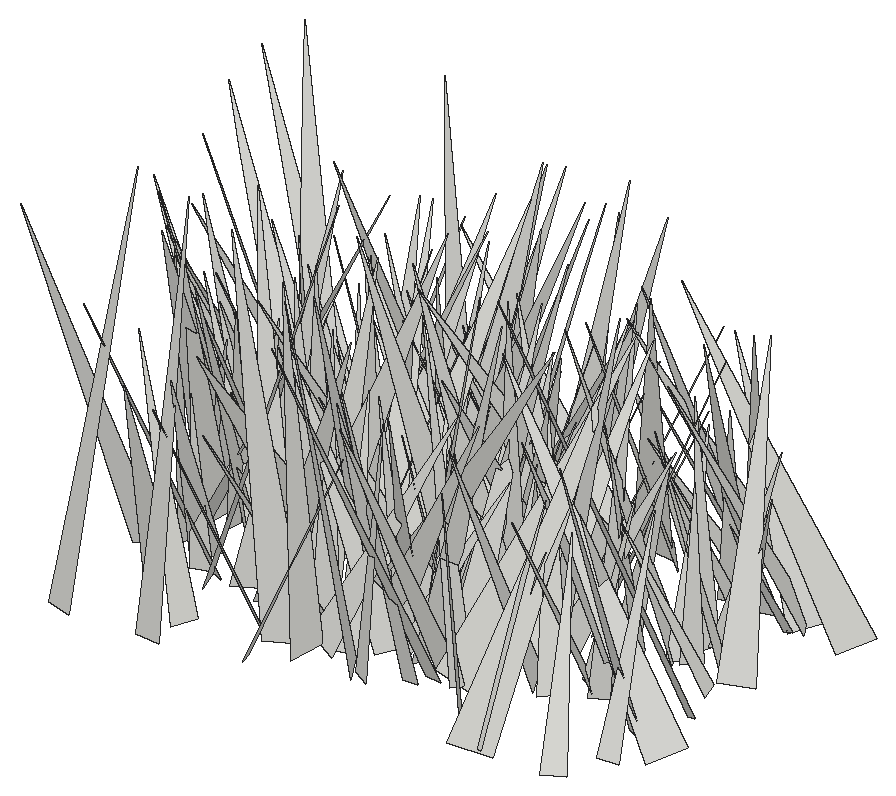
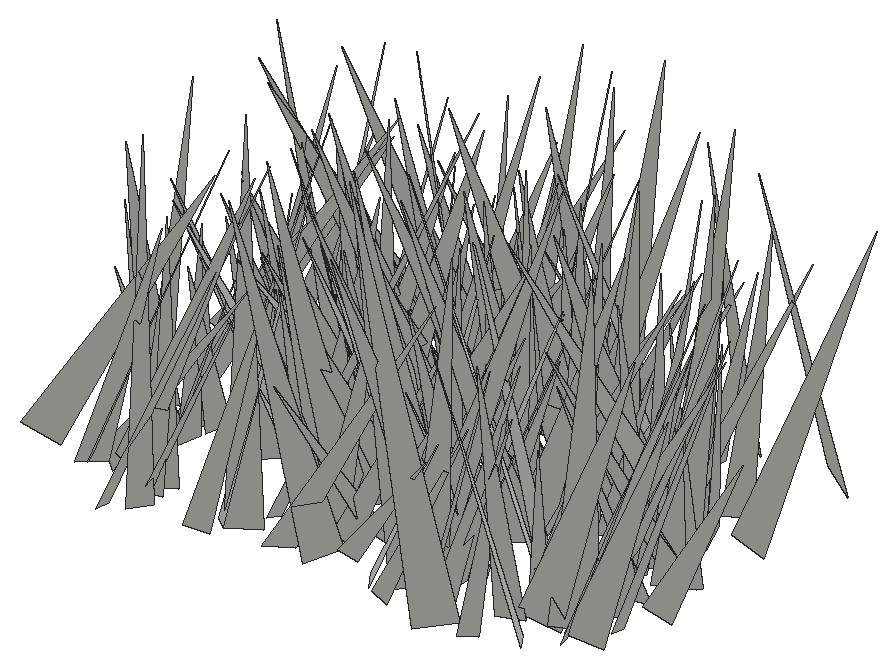
# SketchUp Ruby script. Lengths in inches.
U = 1.inch
M = Sketchup.active_model
def pt(a) = Geom::Point3d.new(a.map { |v| v * U })
def face(e, loops, mat)
  f = e.add_face(loops[0].map { |a| pt(a) })
  loops[1..].each { |l| e.add_face(l.map { |a| pt(a) }).erase! }
  f.material = f.back_material = mat if mat
  f
end
# faces: each face lists its corners as indices into pts; further lists are holes
def faces(e, pts, list, mat = nil) = list.each { |f| face(e, (f[0].is_a?(Array) ? f : [f]).map { |l| l.map { |i| pts[i] } }, mat) }
# xy, xz, yz: faces in a plane at the given z, y or x. An outline is a flat list of corners, or four numbers for a rectangle; further outlines are holes
def ring(l) = l.size == 4 ? [[l[0], l[1]], [l[2], l[1]], [l[2], l[3]], [l[0], l[3]]] : l.each_slice(2).to_a
def flat(e, list, mat, &to3) = list.each { |f| face(e, (f[0].is_a?(Array) ? f : [f]).map { |l| ring(l).map { |u, v| to3.(u, v) } }, mat) }
def xy(e, z, list, mat = nil) = flat(e, list, mat) { |x, y| [x, y, z] }
def xz(e, y, list, mat = nil) = flat(e, list, mat) { |x, z| [x, y, z] }
def yz(e, x, list, mat = nil) = flat(e, list, mat) { |y, z| [x, y, z] }
def lines(e, pts, list) = list.each { |a, b| e.add_line(pt(pts[a]), pt(pts[b])) }
# prism: a flat outline (further loops are holes) pulled along v
def prism(e, loops, v, mat = nil)
  f = face(e, loops, mat); d = Geom::Vector3d.new(v.map { |x| x * U })
  f.pushpull(f.normal.samedirection?(d) ? d.length : -d.length)
end
def box(e, o, s, mat = nil) = prism(e, [[o, [o[0] + s[0], o[1], o[2]], [o[0] + s[0], o[1] + s[1], o[2]], [o[0], o[1] + s[1], o[2]]]], [0, 0, s[2]], mat)
def at(x, y, z, deg = 0) = Geom::Transformation.translation(pt([x, y, z])) * Geom::Transformation.rotation(ORIGIN, Z_AXIS, deg.degrees)
def axes(o, x, y, z) = Geom::Transformation.new([*x, 0, *y, 0, *z, 0, *pt(o).to_a, 1])
def part(name) = M.definitions.add(name)
# library, detail: a bought-in or finely detailed component or shape, given as its bounding box
def library(name, o, s) = part(name).tap { |d| box(d.entities, o, s) }
def detail(e, o, s) = box(e.add_group.entities, o, s)
def put(e, d, t, mat = nil) = e.add_instance(d, t).tap { |i| i.material = mat if mat }
def group(e, t, mat = nil) = e.add_group.tap { |g| g.transformation = t; g.material = mat if mat }.entities
root = M.entities
c1 = part("fur_instance\#9")
p = [[0.8125,0,1.79],[0.67,-0.02,1.48],[0,-0.11,0],[0,0.11,0]]
faces(c1.entities,p,[[0,1,2,3]])
put(root,c1,axes([458.25,101.48,-21.86],[3.84252,-3.67557,0.42443],[-3.56655,-3.84235,-0.9854],[-0.98471,-0.42605,5.2253]))
put(root,c1,axes([461.14,97.17,-21.66],[2.8075,7.47142,1.47372],[7.21104,-3.11318,2.04573],[-2.44844,-0.60171,7.71486]))
put(root,c1,axes([467.92,100.34,-21.86],[-6.16765,-3.82155,1.90605],[-3.98751,6.35208,-0.16723],[1.52874,1.15063,7.2537]))
put(root,c1,axes([473.27,99.74,-21.86],[-3.53133,-2.30027,1.49102],[-2.55807,3.63918,-0.44418],[0.98523,1.20406,4.19097]))
put(root,c1,axes([463.6,100.56,-21.86],[-3.04212,-3.44962,0.11938],[-3.35963,2.92271,-1.15727],[-0.79185,0.85236,4.45141]))
put(root,c1,axes([457.1,97.23,-21.86],[3.59561,7.30217,1.1805],[7.09033,-3.77639,1.76345],[-2.10771,-0.24675,7.94609]))
put(root,c1,axes([464.9,100.28,-21.86],[1.59006,-7.38899,3.46765],[-7.94346,-2.21328,-1.07372],[-1.87702,3.10714,7.48148]))
put(root,c1,axes([461.2,99.19,-21.86],[-5.26641,1.25593,0.32091],[1.22212,5.2582,-0.5227],[0.43216,0.43524,5.3888]))
put(root,c1,axes([478.27,98.73,-21.86],[-2.52047,3.62206,0.22803],[3.61381,2.53037,-0.24846],[0.33426,-0.04477,4.40572]))
put(root,c1,axes([464.5,98.53,-21.86],[4.05537,2.07279,0.17475],[1.9711,-3.95155,1.12829],[-0.66463,0.92835,4.41242]))
put(root,c1,axes([465.9,100.24,-21.86],[-6.94561,0.7265,2.56424],[0.79665,7.39636,0.06233],[2.54332,-0.33278,6.98322]))
put(root,c1,axes([470.83,101.21,-21.66],[-3.56669,-5.90918,0.59479],[-5.71236,3.22345,-2.22975],[-1.62517,1.63841,6.53207]))
put(root,c1,axes([474.76,98.625,-21.86],[1.79845,4.31058,0.12569],[4.2592,-1.79684,0.67963],[-0.67534,0.14702,4.621]))
put(root,c1,axes([470.71,102.27,-21.86],[-0.3519,-5.66898,0.64957],[-5.59847,0.21723,-1.13712],[-1.1029,0.70611,5.5649]))
put(root,c1,axes([468.54,99.99,-21.86],[2.39277,4.07076,1.54907],[4.21231,-2.6123,0.35825],[-1.10775,-1.14055,4.7083]))
put(root,c1,axes([466.13,101.58,-21.86],[-1.49578,-4.28811,0.26565],[-3.87905,1.22698,-2.03551],[-1.84701,0.89578,4.0598]))
put(root,c1,axes([474.94,104.88,-21.86],[-3.72735,-5.65721,0.3773],[-4.71825,3.34531,3.54775],[3.14396,-1.68653,5.77153]))
put(root,c1,axes([470.11,100.81,-21.86],[-2.85535,-4.62994,1.75531],[-4.89429,2.33192,-1.81068],[-0.75056,2.40755,5.12941]))
put(root,c1,axes([458.92,103.32,-21.86],[4.17409,-3.35782,0.27535],[-3.2273,-4.11088,-1.20788],[-0.96712,-0.77425,5.2191]))
put(root,c1,axes([467.72,102.88,-21.86],[0.67121,-5.58126,0.90748],[-5.6399,-0.72653,-0.2969],[-0.40679,0.86382,5.61363]))
put(root,c1,axes([466.71,103.46,-21.86],[-1.5232,-7.73744,1.34983],[-7.81047,1.63722,0.57115],[0.82858,1.20901,7.86523]))
put(root,c1,axes([459.89,102.59,-21.86],[-3.27123,-4.88451,0.3113],[-4.82797,3.15879,-1.17003],[-0.80376,0.90546,5.76111]))
put(root,c1,axes([462.75,102.37,-21.86],[5.42547,-4.53511,0.52895],[-4.56014,-5.3411,0.98008],[0.2284,1.09004,7.00303]))
put(root,c1,axes([467.49,104.29,-21.66],[-1.30326,-6.4856,0.41929],[-6.05179,1.36694,2.33336],[2.36951,-0.07596,6.19006]))
put(root,c1,axes([473.47,103.78,-21.86],[-5.10979,-2.8974,1.28802],[-2.4355,5.15064,1.92434],[2.03034,-1.11347,5.54994]))
put(root,c1,axes([478.84,102.74,-21.86],[-2.84226,-5.05917,1.08036],[-5.16298,2.85167,-0.22901],[0.32566,1.05526,5.79838]))
put(root,c1,axes([474.01,100.5,-21.86],[0.88242,4.55252,0.64978],[4.54635,-0.76413,-0.82042],[0.6916,-0.78549,4.5641]))
put(root,c1,axes([462.64,105.77,-21.66],[6.08431,-4.17162,0.61258],[-3.3903,-5.47976,-3.64343],[-2.50671,-2.71408,6.41457]))
put(root,c1,axes([465.93,100.97,-21.86],[1.55014,5.60518,1.20615],[5.3228,-0.94254,-2.46072],[2.13086,-1.72318,5.26933]))
put(root,c1,axes([472.63,102.54,-21.66],[3.70621,1.73352,0.50221],[1.78343,-3.34171,-1.62653],[0.27688,-1.67963,3.75439]))
put(root,c1,axes([468.23,102.23,-21.86],[-3.70212,4.89762,1.86065],[5.19102,3.12087,2.11373],[-0.70854,-2.72541,5.76407]))
put(root,c1,axes([456.65,102.88,-21.86],[-0.79345,-6.87819,1.77521],[-6.83318,0.25089,-2.08208],[-1.94125,1.92821,6.60333]))
put(root,c1,axes([459.3,102.52,-21.86],[1.04159,-3.44564,1.2731],[-3.64709,-1.12789,-0.06873],[-0.4381,1.19732,3.59897]))
put(root,c1,axes([467.25,102.83,-21.66],[3.81653,-4.78014,0.36891],[-4.62204,-3.54318,1.90641],[1.2738,1.46558,5.81217]))
put(root,c1,axes([467.17,101.08,-21.86],[-0.50295,4.78104,0.71911],[4.81704,0.43358,0.48636],[-0.41423,-0.76294,4.78276]))
put(root,c1,axes([474.8,98.32,-21.86],[-6.00676,5.62271,0.83771],[4.81686,5.68135,-3.59416],[3.01902,2.12255,7.40122]))
put(root,c1,axes([479.12,100.74,-21.86],[0.03105,4.61747,0.04613],[4.59439,-0.03553,0.46309],[-0.46341,-0.04278,4.59429]))
put(root,c1,axes([469.55,104.09,-21.86],[3.26712,2.26093,2.86418],[3.20778,-3.61207,-0.80776],[-1.73938,-2.41465,3.89016]))
put(root,c1,axes([468.51,102.69,-21.86],[-0.19493,4.51759,1.73565],[4.75586,-0.14282,0.90585],[-0.89608,-1.74071,4.43013]))
put(root,c1,axes([470.55,103.74,-21.86],[-2.5232,4.5633,1.53247],[4.25008,1.29942,3.12842],[-2.26029,-2.65076,4.17172]))
put(root,c1,axes([466.51,103.35,-21.66],[6.17977,-5.38552,0.13557],[-5.06059,-5.73249,2.95646],[1.84733,2.31224,7.64543]))
put(root,c1,axes([468.4375,102.42,-21.86],[1.55212,3.88569,0.28277],[3.69063,-1.36892,-1.44671],[1.24813,-0.78428,3.92616]))
put(root,c1,axes([469.63,102.4375,-21.86],[6.54484,-1.1484,2.12677],[-1.53141,-6.71985,1.08414],[-1.86996,1.48383,6.55579]))
put(root,c1,axes([480.52,102.31,-21.86],[-3.77529,6.85051,0.02559],[5.94676,3.26269,3.89536],[-3.40091,-1.89957,6.78296]))
put(root,c1,axes([464.61,102.875,-21.86],[-0.09344,5.23116,1.72248],[5.50098,0.0052,0.28262],[-0.26677,-1.725,5.22436]))
put(root,c1,axes([468.16,103.8,-21.86],[6.04593,4.4435,2.18806],[4.86244,-5.98205,-1.28733],[-0.94282,-2.35709,7.39194]))
put(root,c1,axes([463.61,103.91,-21.86],[-3.32714,-4.87132,0.7615],[-4.7527,2.92423,-2.05917],[-1.31203,1.7603,5.52806]))
put(root,c1,axes([476.75,104.84,-21.86],[-1.00098,-5.50903,0.83943],[-5.47181,0.81017,-1.20786],[-1.05515,1.02481,5.46739]))
put(root,c1,axes([471.96,101.46,-21.66],[-6.70082,0.16595,0.10129],[0.12128,6.29761,-2.29436],[0.15195,2.29157,6.29797]))
put(root,c1,axes([456.65,107.05,-21.66],[7.11754,-4.23376,0.53848],[-3.90576,-6.88369,-2.49681],[-1.7204,-1.88792,7.89621]))
put(root,c1,axes([471.64,101.5,-21.66],[-0.75445,7.6495,1.46212],[7.18414,1.25072,-2.83648],[3.00677,-1.06897,7.14412]))
put(root,c1,axes([476.84,105.47,-21.66],[3.36953,-3.09183,0.80409],[-2.80421,-3.42236,-1.4084],[-1.53048,-0.53643,4.35081]))
put(root,c1,axes([457.4,105.68,-21.86],[6.33398,-2.31725,1.64534],[-1.9481,-6.46653,-1.60778],[-2.06922,-1.00519,6.55011]))
put(root,c1,axes([458.57,106.36,-21.86],[6.05103,1.03829,2.78411],[2.19851,-5.8136,-2.61017],[-1.99898,-3.2509,5.55698]))
put(root,c1,axes([460.2,101.77,-21.66],[6.70956,3.50603,1.11128],[3.28027,-6.75003,1.49074],[-1.66343,0.8308,7.42214]))
put(root,c1,axes([472.53,102.65,-21.86],[0.12612,4.07155,0.3622],[4.08216,-0.1442,0.19951],[-0.2114,-0.35539,4.06861]))
put(root,c1,axes([474.62,103.24,-21.86],[-4.08375,3.22336,1.0157],[3.24667,4.18417,-0.22495],[0.93853,-0.4488,5.19774]))
put(root,c1,axes([462.22,103.21,-21.86],[-1.69454,7.12423,1.83382],[7.32335,1.45532,1.11334],[-0.69716,-2.02889,7.23786]))
put(root,c1,axes([460.97,105.69,-21.66],[-3.68775,-0.43694,1.2324],[0.03671,3.65173,1.40455],[1.30705,-1.33536,3.43768]))
put(root,c1,axes([468.62,106.24,-21.86],[-7.9399,0.37328,2.34081],[0.92834,8.01881,1.87016],[2.18103,-2.05426,7.72553]))
put(root,c1,axes([463.38,104.08,-21.86],[-3.27295,5.40819,2.7555],[5.57889,3.91368,-1.05481],[2.39109,-1.7286,6.23283]))
put(root,c1,axes([473.25,104.74,-21.86],[-2.12698,-6.60371,3.80122],[-7.1046,3.14508,1.48842],[2.75369,3.0136,6.77625]))
put(root,c1,axes([458.24,106.06,-21.86],[5.00192,-1.81934,1.03799],[-1.65,-5.07776,-0.94895],[-1.29032,-0.55947,5.23724]))
put(root,c1,axes([457.76,103.48,-21.66],[-5.24858,-0.93793,1.2858],[-1.33069,5.01688,-1.77222],[0.87308,2.00792,5.02857]))
put(root,c1,axes([462.75,104.125,-21.66],[5.54256,-5.39998,2.31392],[-5.86744,-4.92827,2.55329],[0.29519,3.43313,7.30483]))
put(root,c1,axes([468.51,103.62,-21.86],[-1.50833,4.20798,0.27956],[4.21722,1.50618,0.08227],[0.01672,-0.29093,4.46939]))
put(root,c1,axes([464.42,108.38,-21.66],[-5.86145,-3.99032,0.23805],[-3.68658,5.55942,2.41617],[1.54546,-1.87245,6.66644]))
put(root,c1,axes([462.1875,105.31,-21.86],[1.65081,-5.08845,2.41171],[-5.51574,-1.96719,-0.37505],[-1.13372,2.16141,5.33637]))
put(root,c1,axes([479.47,105.03,-21.86],[-5.76145,-5.93812,0.42997],[-5.44241,5.01036,-3.73055],[-2.41379,2.87671,7.38502]))
put(root,c1,axes([459.67,105.48,-21.86],[-5.88104,-3.53705,0.94417],[-3.64814,5.81133,-0.9531],[0.30541,1.30636,6.79625]))
put(root,c1,axes([468.73,103.02,-21.66],[-1.68385,4.77561,0.18208],[4.53538,1.65768,-1.53538],[1.50664,0.34725,4.82539]))
put(root,c1,axes([470.98,105.65,-21.86],[-0.03383,-6.90938,2.82252],[-7.12958,-0.80509,-2.05628],[-2.20801,2.70547,6.5964]))
put(root,c1,axes([456.03,106.71,-21.66],[-0.42992,-4.68733,0.89248],[-4.33891,0.75688,1.88505],[1.98531,0.63912,4.31306]))
put(root,c1,axes([461.78,106.16,-21.86],[2.04038,-5.82637,1.87095],[-6.1057,-2.07021,0.21174],[-0.4092,1.83789,6.16967]))
put(root,c1,axes([463.15,106.35,-21.66],[-3.41079,-4.86692,0.40111],[-4.72199,3.16213,-1.78467],[-1.24525,1.33989,5.66881]))
put(root,c1,axes([470.875,102.72,-21.66],[-5.5806,3.5391,0.90465],[3.04631,5.42049,-2.4135],[2.01583,1.60617,6.15169]))
put(root,c1,axes([475.0625,104.67,-21.86],[1.48501,3.27806,0.44782],[3.28348,-1.52047,0.24164],[-0.40618,-0.30651,3.59062]))
put(root,c1,axes([461.37,102.6,-21.86],[-6.96616,2.88196,1.8212],[2.05018,6.85162,-3.00033],[2.72382,2.21349,6.91601]))
put(root,c1,axes([458.64,106.31,-21.86],[2.66304,-4.00114,1.09323],[-4.14622,-2.60379,0.57024],[-0.11461,1.22768,4.77239]))
put(root,c1,axes([463.79,106.36,-21.86],[-0.58668,-6.43534,2.37936],[-6.81319,0.82822,0.56013],[0.80964,2.30643,6.43771]))
put(root,c1,axes([459.84,105.35,-21.86],[-4.98087,1.16288,0.32288],[1.15979,4.99131,-0.08543],[0.33384,0.00996,5.1141]))
put(root,c1,axes([470.3,109.09,-21.66],[3.62515,-5.36286,0.15908],[-5.03579,-3.46731,-2.13211],[-1.85105,-1.06996,6.11196]))
put(root,c1,axes([470.2,106.54,-21.86],[0.12589,-6.48138,2.39431],[-6.90548,-0.03647,0.26437],[0.23531,2.39734,6.47721]))
put(root,c1,axes([478.76,106.93,-21.86],[-3.57731,-0.93265,0.01118],[-0.92223,3.54345,0.51048],[0.1395,-0.49118,3.66148]))
put(root,c1,axes([466.12,103.71,-21.86],[-5.45003,5.37343,0.92209],[5.18096,5.51046,-1.48977],[1.69756,0.43353,7.50714]))
put(root,c1,axes([469.28,104.88,-21.66],[7.05742,-1.09775,2.22467],[-1.64487,-7.09246,1.71837],[-1.85705,2.1103,6.93249]))
put(root,c1,axes([464.99,103.97,-21.66],[4.59925,2.87418,0.36346],[2.61006,-4.40682,1.82035],[-1.25721,1.36572,5.10885]))
put(root,c1,axes([463.28,106.78,-21.66],[-4.72001,4.32069,1.36462],[4.52973,4.45158,1.57294],[-0.11027,-2.07946,6.20264]))
put(root,c1,axes([475.36,107.23,-21.86],[-4.36965,-1.59831,1.51111],[-1.58231,4.61869,0.30967],[1.52785,0.21216,4.64247]))
put(root,c1,axes([472.71,106.48,-21.86],[0.36945,4.73641,1.83647],[4.53767,0.52011,-2.25427],[2.28381,-1.79961,4.18191]))
put(root,c1,axes([458.46,107.23,-21.86],[-6.02827,1.48886,1.73676],[1.72693,6.17226,0.7029],[1.50026,-1.12234,6.1695]))
put(root,c1,axes([464.27,106.85,-21.86],[-4.31803,3.62073,2.04082],[3.93255,4.51165,0.31626],[1.34522,-1.56695,5.62628]))
put(root,c1,axes([463.55,108.02,-21.86],[5.97247,-1.71505,1.0533],[-1.60325,-6.04797,-0.7569],[-1.21673,-0.44932,6.16757]))
put(root,c1,axes([457.55,104.45,-21.86],[7.33228,1.89466,0.16833],[1.78282,-7.07911,2.02191],[-0.66303,1.91751,7.29821]))
put(root,c1,axes([472.62,104.52,-21.66],[-1.93845,6.02083,0.54238],[5.77969,2.01278,-1.68701],[1.77192,0.02133,6.09606]))
put(root,c1,axes([469.87,107,-21.86],[-3.1989,2.68909,0.37978],[2.66785,3.00183,1.21655],[-0.50792,-1.16886,3.99802]))
put(root,c1,axes([476.22,108.3,-21.86],[-6.24569,-2.79636,0.92417],[-2.76847,6.31368,0.39421],[1.00464,0.01396,6.83176]))
put(root,c1,axes([476.06,104.05,-21.86],[2.20032,6.76237,0.49836],[6.15454,-2.21163,2.83722],[-2.84601,0.44546,6.52083]))
put(root,c1,axes([468.76,106.53,-21.66],[-3.29072,5.65648,0.59206],[5.32719,2.82602,2.60955],[-1.99181,-1.7869,6.00123]))
put(root,c1,axes([468.65,109.02,-21.66],[1.7793,-6.50243,0.4842],[-6.28195,-1.575,1.93351],[1.74732,0.95904,6.45825]))
put(root,c1,axes([465.34,104.82,-21.86],[-0.97355,8.05143,1.14446],[7.84551,1.23329,-2.00251],[2.14086,-0.85824,7.85896]))
put(root,c1,axes([464.37,107.35,-21.86],[-3.83694,1.86592,0.39498],[1.90547,3.78872,0.61201],[0.08273,-0.72368,4.22246]))
put(root,c1,axes([470.21,105.38,-21.86],[4.5765,3.32185,0.66717],[3.07667,-4.544,1.52],[-1.41913,0.86116,5.4469]))
put(root,c1,axes([472.44,106.97,-21.66],[-2.33709,5.71521,1.48586],[5.84354,2.00796,1.46781],[-0.85111,-1.90732,5.99759]))
put(root,c1,axes([471.05,111.63,-21.86],[-7.67561,-3.02253,0.64542],[-2.50236,7.09168,3.4516],[1.81396,-3.00659,7.49247]))
put(root,c1,axes([468.56,108.5,-21.66],[3.57739,2.98141,0.96801],[3.07785,-3.06266,-1.94177],[0.59384,-2.08684,4.23274]))
put(root,c1,axes([467.98,107.96,-21.86],[3.19259,1.80159,0.09548],[1.75198,-3.04965,-1.03811],[0.43061,-0.9494,3.51578]))
put(root,c1,axes([457.11,109.75,-21.86],[-4.32761,-0.50237,2.11035],[0.41917,4.42689,1.9134],[2.12844,-1.89326,3.91401]))
put(root,c1,axes([457.63,109.63,-21.86],[-5.22696,-1.19875,0.73288],[-0.94186,5.08442,1.59898],[1.04259,-1.41663,5.11873]))
put(root,c1,axes([471.87,104.67,-21.66],[4.84887,3.21318,0.05137],[2.84684,-4.33809,2.62966],[-1.49084,2.16682,5.18854]))
put(root,c1,axes([477.08,108.04,-21.86],[-2.3678,2.48019,1.72309],[2.76192,2.66404,-0.03926],[1.22155,-1.2159,3.42875]))
put(root,c1,axes([473.83,108.51,-21.86],[1.56073,-4.1385,0.9971],[-4.17951,-1.28812,1.1957],[0.80812,1.33073,4.25833]))
put(root,c1,axes([457.1,106.37,-21.66],[0.04423,5.29855,0.55334],[5.02486,0.14232,-1.76445],[1.76963,-0.53655,4.99632]))
put(root,c1,axes([467.75,107.28,-21.86],[4.89085,0.64493,0.58721],[0.56841,-4.89366,0.64042],[-0.66156,0.56328,4.89144]))
put(root,c1,axes([465.27,107.3,-21.66],[-5.24793,-3.08562,0.82091],[-3.15493,4.76816,-2.24651],[-0.49124,2.34081,5.65818]))
put(root,c1,axes([469.05,107.61,-21.86],[-2.42701,4.03219,1.90827],[4.11447,2.86278,-0.81615],[1.72373,-1.15601,4.63496]))
put(root,c1,axes([458.76,109.81,-21.66],[-2.19806,-5.17129,0.07017],[-4.98418,2.09779,-1.52836],[-1.38027,0.66005,5.4072]))
put(root,c1,axes([458.02,109.41,-21.86],[-3.08221,-2.2445,0.63722],[-2.14243,3.14072,0.69983],[0.92405,-0.20483,3.74807]))
put(root,c1,axes([466.16,108.65,-21.86],[-4.51711,1.79985,0.33219],[1.82954,4.41557,0.95372],[-0.05124,-1.00862,4.76803]))
put(root,c1,axes([466.82,106.83,-21.86],[4.77639,3.07128,1.21309],[2.81816,-4.90311,1.31748],[-1.72115,0.49496,5.52367]))
put(root,c1,axes([460.77,107.34,-21.66],[2.36274,4.29484,1.97791],[3.91667,-3.01643,1.87116],[-2.64906,-0.62918,4.53067]))
put(root,c1,axes([460.49,109.29,-21.86],[6.75177,1.95337,0.7466],[2.07523,-6.56983,-1.57805],[-0.25785,-1.72661,6.84922]))
put(root,c1,axes([456.2,110.79,-21.66],[-5.34659,-1.99732,0.9572],[-1.60106,5.21354,1.93576],[1.5304,-1.52357,5.36919]))
put(root,c1,axes([465.65,107.08,-21.66],[7.81962,-2.04899,1.63917],[-2.46618,-7.49875,2.3913],[-0.8962,2.75717,7.72182]))
put(root,c1,axes([478.02,108.625,-21.86],[-4.15206,-1.52587,0.16301],[-1.50616,3.96212,-1.27574],[-0.29385,1.25209,4.2356]))
put(root,c1,axes([464.47,109.9375,-21.86],[5.48977,-0.87036,1.92832],[-0.64898,-5.79667,-0.76876],[-2.01365,-0.50463,5.50492]))
put(root,c1,axes([472.66,108.25,-21.86],[4.47916,2.33614,0.04477],[2.33654,-4.47877,-0.05982],[-0.01203,-0.07375,5.05142]))
put(root,c1,axes([464.8,112.3,-21.86],[-3.43989,-5.36661,0.1848],[-4.97328,3.26677,2.29397],[2.02515,-1.09328,5.94736]))
put(root,c1,axes([472.86,107.96,-21.86],[5.67742,2.27779,0.25934],[2.25803,-5.67581,0.41845],[-0.39608,0.29237,6.10297]))
put(root,c1,axes([456.96,108.38,-21.86],[1.35315,4.35582,0.79538],[4.34518,-1.14634,-1.11449],[0.85157,-1.07217,4.42291]))
put(root,c1,axes([462.74,107.78,-21.66],[-0.40245,7.17423,1.83924],[7.10701,0.89237,-1.92572],[2.08393,-1.65784,6.92265]))
put(root,c1,axes([460.3,109.89,-21.66],[6.41393,4.45568,0.74677],[4.39818,-5.86174,-2.80093],[1.0328,-2.70854,7.29015]))
put(root,c1,axes([476.55,107.92,-21.86],[-3.56654,2.39752,0.7344],[2.22273,3.6139,-1.00345],[1.16058,0.44646,4.17868]))
put(root,c1,axes([479.29,107.81,-21.86],[-2.49742,5.95651,1.04282],[6.02179,2.55284,-0.16018],[0.55273,-0.89868,6.45689]))
put(root,c1,axes([457.24,112.55,-21.66],[-5.6995,-3.45113,0.56108],[-3.05969,5.44221,2.39374],[1.69215,-1.78365,6.21808]))
put(root,c1,axes([476.83,109.27,-21.86],[-4.53937,1.16522,1.40638],[1.15678,4.75002,-0.2018],[1.41333,-0.14527,4.6822]))
put(root,c1,axes([467.91,107.99,-21.86],[6.07013,4.91373,1.22638],[4.90353,-6.18107,0.495],[-1.26656,-0.38061,7.79399]))
put(root,c1,axes([464.25,111.68,-21.66],[-0.98604,-7.77609,1.14314],[-7.75331,0.77346,-1.42635],[-1.28859,1.29646,7.70749]))
put(root,c1,axes([476.89,111.48,-21.66],[4.69242,0.16576,0.10905],[0.19618,-4.2622,-1.96297],[-0.02968,-1.96577,4.26532]))
put(root,c1,axes([471.76,107.82,-21.86],[5.6659,3.07924,0.02777],[3.03508,-5.59401,1.03936],[-0.52039,0.90013,6.36426]))
put(root,c1,axes([455.8,109.04,-21.66],[-1.87407,5.07403,0.37598],[4.58214,1.50899,2.47512],[-2.21159,-1.17322,4.80954]))
put(root,c1,axes([467.35,108.48,-21.86],[5.97099,-0.01983,0.33196],[-0.11666,-5.7151,1.75709],[-0.31141,1.76085,5.70664]))
put(root,c1,axes([478.56,112.65,-21.66],[-5.31145,-3.30369,0.30508],[-3.10318,5.15062,1.7494],[1.17379,-1.33255,6.00546]))
put(root,c1,axes([466.17,108.37,-21.66],[6.99612,0.8962,1.32294],[0.53893,-6.91662,1.83548],[-1.5043,1.69005,6.81028]))
put(root,c1,axes([475.62,113.125,-21.86],[-0.94018,-7.50089,0.47804],[-7.29693,1.02641,1.75419],[1.80188,0.24278,7.35324]))
put(root,c1,axes([468.71,110.62,-21.86],[-2.71564,-2.49022,0.0198],[-2.39499,2.6036,-1.03032],[-0.68234,0.77224,3.53756]))
put(root,c1,axes([458.17,110.61,-21.66],[-4.54723,-4.75664,0.92618],[-4.80738,4.26788,-1.68375],[-0.61038,1.82216,6.36144]))
put(root,c1,axes([464.98,108.95,-21.86],[2.99625,3.60782,0.19235],[3.59342,-3.00177,0.328],[-0.37513,0.06212,4.67828]))
put(root,c1,axes([468.07,111.46,-21.86],[0.12283,-4.44104,1.09952],[-4.1986,-0.54638,-1.73783],[-1.81756,0.96203,4.08875]))
put(root,c1,axes([464.7,108.84,-21.86],[4.91626,-1.03874,2.91243],[-2.03601,-5.20453,1.58061],[-2.3272,2.35896,4.76972]))
put(root,c1,axes([475.92,112.1,-21.86],[-3.49973,-1.74713,0.54329],[-1.50598,3.41664,1.28623],[1.03907,-0.93268,3.69408]))
put(root,c1,axes([477.07,109.61,-21.86],[3.51726,-1.23078,1.44078],[-1.67757,-3.4351,1.16087],[-0.88116,1.62697,3.54095]))
put(root,c1,axes([469.24,110.59,-21.86],[1.69917,-3.99461,2.49122],[-4.30676,-2.38859,-0.89256],[-1.90128,1.84064,4.24822]))
put(root,c1,axes([471.13,113.25,-21.66],[1.38948,-7.3294,0.52561],[-7.22169,-1.26322,1.47599],[1.35779,0.7818,7.31247]))
put(root,c1,axes([469.12,111.49,-21.86],[3.70766,-2.56946,0.56874],[-2.62102,-3.69364,0.39947],[-0.23628,0.65362,4.49325]))
put(root,c1,axes([472.05,113.41,-21.66],[-4.28945,-4.51982,0.83876],[-4.25056,4.33652,1.63064],[1.75072,-0.54543,6.01408]))
put(root,c1,axes([459.84,111.11,-21.86],[-4.13289,0.76106,0.51137],[0.79822,4.14817,0.27763],[0.45116,-0.36746,4.1932]))
put(root,c1,axes([462.58,110.16,-21.86],[3.48298,2.03603,0.22687],[2.02285,-3.48877,0.25421],[-0.32396,0.10555,4.02641]))
put(root,c1,axes([469.55,109.32,-21.86],[-6.57541,3.25527,2.97746],[2.73361,7.20101,-1.83599],[3.46258,0.49673,7.10365]))
put(root,c1,axes([460.27,110.15,-21.86],[-3.61922,1.27993,0.57976],[1.16278,3.62754,-0.74965],[0.78884,0.52519,3.76496]))
put(root,c1,axes([464.37,110.65,-21.66],[-0.74897,7.24815,2.93985],[7.55595,1.43371,-1.60981],[2.0214,-2.6736,7.1067]))
put(root,c1,axes([475.39,112.4375,-21.86],[1.74282,-4.6233,0.69197],[-4.67126,-1.6936,0.44965],[0.18179,0.80496,4.92038]))
put(root,c1,axes([477.14,112.29,-21.66],[-2.01567,-6.30283,1.43527],[-6.28052,1.55369,-1.99742],[-1.52993,1.92587,6.30864]))
put(root,c1,axes([467.27,110.52,-21.86],[-1.27036,4.00789,0.19304],[3.62684,1.0603,1.85365],[-1.71652,-0.72583,3.77372]))
put(root,c1,axes([478.28,111.98,-21.86],[-2.89235,-4.23355,0.19447],[-3.82387,2.50545,-2.32964],[-1.82723,1.45817,4.56743]))
put(root,c1,axes([475.41,113.67,-21.86],[-4.08154,-1.42978,0.42723],[-1.12455,3.76494,1.85644],[0.98091,-1.633,3.906]))
put(root,c1,axes([464.11,112.57,-21.86],[4.17452,-5.37379,1.20818],[-5.50555,-4.02647,1.11376],[0.16212,1.6352,6.71296]))
put(root,c1,axes([462.15,113.3,-21.66],[-4.28655,1.17606,1.86698],[1.8295,4.17484,1.57066],[1.23356,-2.10497,4.15821]))
put(root,c1,axes([476.28,114.81,-21.86],[-6.53247,-2.60599,0.49941],[-2.30056,6.22381,2.3844],[1.32211,-2.04617,6.61657]))
put(root,c1,axes([470.23,109.86,-21.86],[2.36714,6.37429,1.14743],[6.22522,-2.57637,1.46983],[-1.78738,-0.5313,6.63886]))
put(root,c1,axes([481.04,112.39,-21.66],[-4.16636,5.9481,1.52453],[5.74666,3.12806,3.50054],[-2.16332,-3.14611,6.36276]))
put(root,c1,axes([462.82,113.32,-21.86],[-3.9819,-2.09854,0.99873],[-1.89028,4.07705,1.03024],[1.35209,-0.4803,4.38155]))
put(root,c1,axes([460.32,114.1,-21.86],[4.10212,-1.60455,0.85508],[-1.23063,-4.00368,-1.60913],[-1.3384,-1.23658,4.10033]))
put(root,c1,axes([475,114.3,-21.66],[6.59264,-0.88288,1.14982],[-0.53637,-6.4595,-1.88457],[-1.3468,-1.74924,6.37893]))
put(root,c1,axes([462.85,111.64,-21.86],[-4.9286,0.63717,0.02707],[0.62924,4.89286,-0.60144],[0.10377,0.59304,4.93308]))
put(root,c1,axes([457.74,111.34,-21.86],[-4.19179,6.94453,1.88873],[7.18228,4.17546,0.58769],[0.45687,-1.92457,8.09026]))
put(root,c1,axes([467.67,110.34,-21.66],[3.89032,1.8987,0.46131],[1.51623,-3.58179,1.95558],[-1.23244,1.58688,3.86204]))
put(root,c1,axes([472.64,114.08,-21.86],[1.77342,-4.13167,0.71101],[-4.001,-1.89854,-1.053],[-1.2523,0.21471,4.37115]))
put(root,c1,axes([469.59,113.21,-21.86],[-6.03456,2.61232,0.13904],[2.52964,5.73798,1.98392],[-0.66667,-1.87372,6.2693]))
put(root,c1,axes([463.98,110.71,-21.86],[6.32729,-2.1008,2.73388],[-3.01636,-6.1404,2.26257],[-1.67006,3.13117,6.27127]))
put(root,c1,axes([478.61,112.52,-21.86],[-4.85696,2.92878,0.85344],[3.03677,4.79447,0.82904],[0.29007,-1.15391,5.61075]))
put(root,c1,axes([464.49,110.99,-21.86],[0.0482,8.00911,1.76337],[7.92916,-0.49572,2.03478],[-2.09374,-1.69294,7.74648]))
put(root,c1,axes([464.51,113.86,-21.86],[-0.70477,-3.63934,0.22038],[-3.52996,0.62491,-0.96896],[-0.91253,0.39339,3.57807]))
put(root,c1,axes([459.98,112.11,-21.86],[-1.16882,5.10436,1.64073],[5.31118,1.33199,-0.3603],[0.7334,-1.51127,5.22406]))
put(root,c1,axes([456.88,111.81,-21.86],[-3.24359,5.98487,0.42852],[5.75195,2.96279,2.1587],[-1.708,-1.38792,6.45597]))
put(root,c1,axes([459,111.73,-21.86],[-3.17251,7.14398,0.8627],[6.87917,2.73438,2.65436],[-2.11131,-1.82544,7.35225]))
put(root,c1,axes([467.05,112.48,-21.66],[-1.66623,3.3763,0.05798],[2.90925,1.40249,1.93607],[-1.71436,-0.9015,3.22914]))
put(root,c1,axes([465.57,113.11,-21.86],[-3.08913,-1.9262,0.20442],[-1.91689,2.98464,-0.84391],[-0.27849,0.82245,3.5413]))
put(root,c1,axes([461.68,114.21,-21.86],[3.88235,-7.18309,1.19208],[-7.15051,-3.50623,2.16032],[1.37403,2.04942,7.87416]))
put(root,c1,axes([467.93,112.77,-21.86],[6.31096,-2.97385,1.65761],[-3.28181,-6.24286,1.29466],[-0.9062,1.89806,6.85536]))
put(root,c1,axes([458.61,113.21,-21.86],[4.70564,3.18962,0.73071],[3.27223,-4.59158,-1.02983],[-0.01227,-1.26267,5.59072]))
